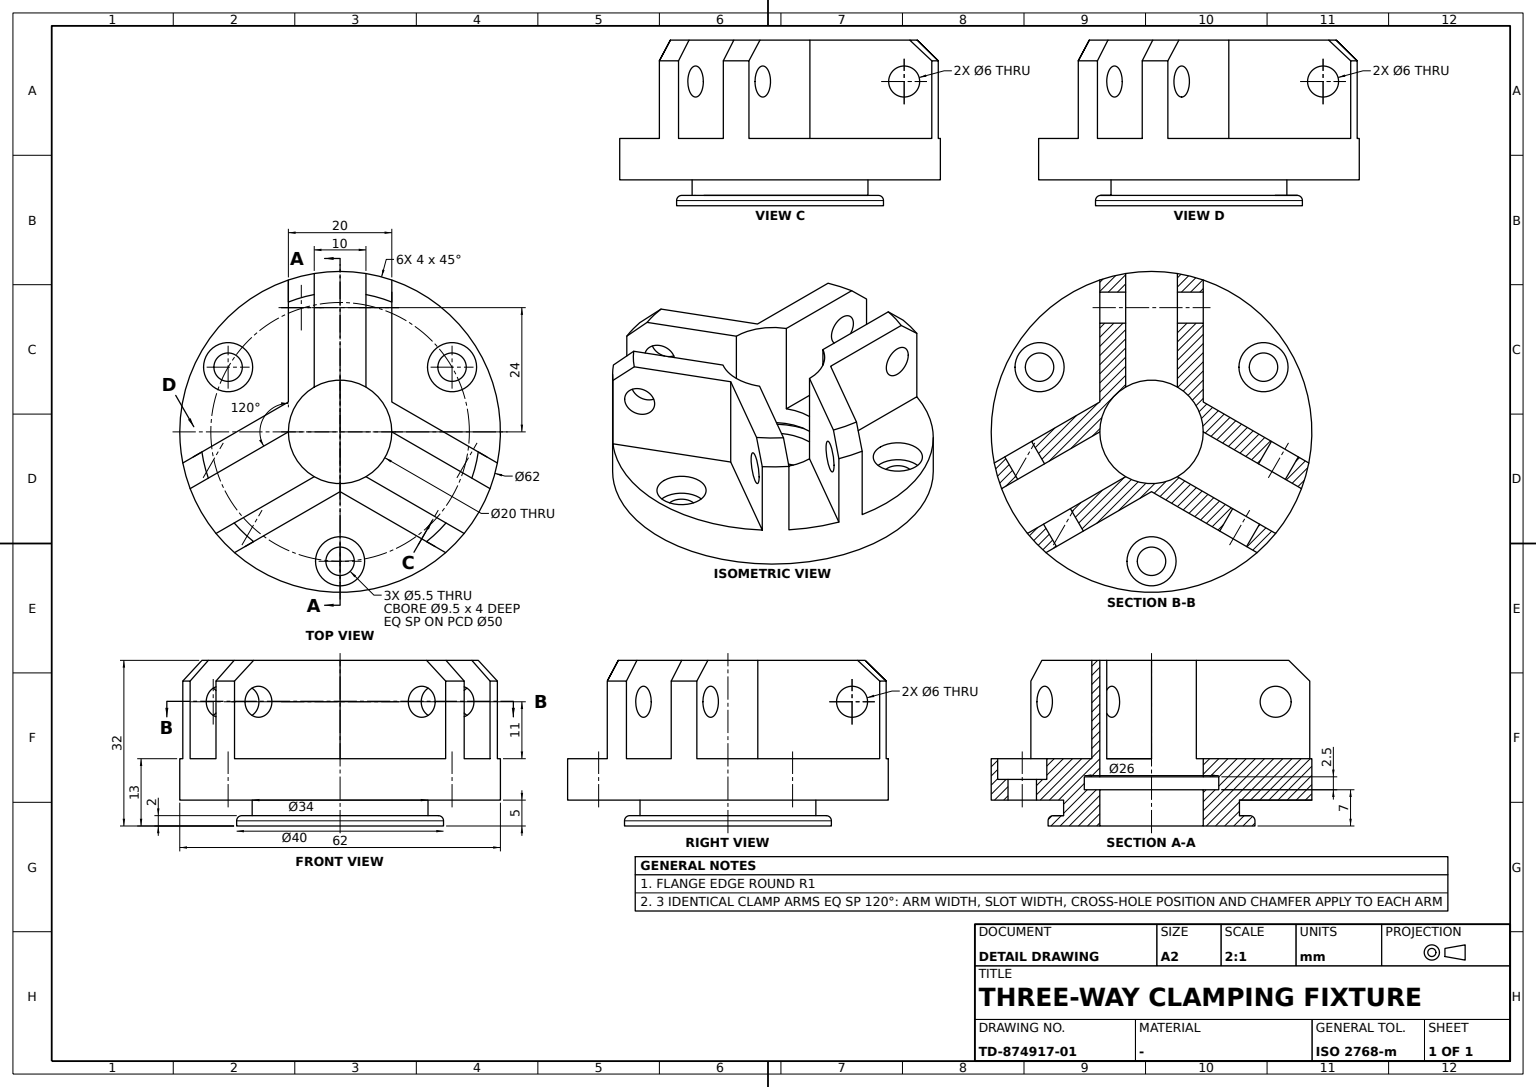
ISO-10303-21;
HEADER;
FILE_DESCRIPTION((''),'2;1');
FILE_NAME('','',(''),(''),'','','');
FILE_SCHEMA(('AUTOMOTIVE_DESIGN'));
ENDSEC;
DATA;
#1=APPLICATION_CONTEXT('');
#2=PRODUCT_CONTEXT('',#1,'mechanical');
#3=PRODUCT('','','',(#2));
#4=PRODUCT_DEFINITION_FORMATION('','',#3);
#5=PRODUCT_DEFINITION_CONTEXT('',#1,'design');
#6=PRODUCT_DEFINITION('','',#4,#5);
#7=PRODUCT_DEFINITION_SHAPE('','',#6);
#8=(LENGTH_UNIT()NAMED_UNIT(*)SI_UNIT(.MILLI.,.METRE.));
#9=(NAMED_UNIT(*)PLANE_ANGLE_UNIT()SI_UNIT($,.RADIAN.));
#10=(NAMED_UNIT(*)SI_UNIT($,.STERADIAN.)SOLID_ANGLE_UNIT());
#11=UNCERTAINTY_MEASURE_WITH_UNIT(LENGTH_MEASURE(0.005),#8,'distance_accuracy_value','');
#12=(GEOMETRIC_REPRESENTATION_CONTEXT(3)GLOBAL_UNCERTAINTY_ASSIGNED_CONTEXT((#11))GLOBAL_UNIT_ASSIGNED_CONTEXT((#8,#9,#10))REPRESENTATION_CONTEXT('',''));
#13=CARTESIAN_POINT('',(-26.400635,12.5,13.));
#14=VERTEX_POINT('',#13);
#15=CARTESIAN_POINT('',(-21.650635,12.5,13.));
#16=DIRECTION('',(0.,0.,-1.));
#17=DIRECTION('',(-1.,0.,0.));
#18=AXIS2_PLACEMENT_3D('',#15,#16,#17);
#19=CIRCLE('',#18,4.75);
#20=EDGE_CURVE('',#14,#14,#19,.T.);
#21=ORIENTED_EDGE('',*,*,#20,.F.);
#22=EDGE_LOOP('',(#21));
#23=FACE_BOUND('',#22,.T.);
#24=CARTESIAN_POINT('',(-26.400635,12.5,9.));
#25=VERTEX_POINT('',#24);
#26=CARTESIAN_POINT('',(-21.650635,12.5,9.));
#27=AXIS2_PLACEMENT_3D('',#26,#16,#17);
#28=CIRCLE('',#27,4.75);
#29=EDGE_CURVE('',#25,#25,#28,.F.);
#30=ORIENTED_EDGE('',*,*,#29,.F.);
#31=EDGE_LOOP('',(#30));
#32=FACE_BOUND('',#31,.T.);
#33=CYLINDRICAL_SURFACE('',#18,4.75);
#34=ADVANCED_FACE('',(#23,#32),#33,.F.);
#35=CARTESIAN_POINT('',(-24.400635,12.5,9.));
#36=VERTEX_POINT('',#35);
#37=CIRCLE('',#27,2.75);
#38=EDGE_CURVE('',#36,#36,#37,.F.);
#39=ORIENTED_EDGE('',*,*,#38,.T.);
#40=EDGE_LOOP('',(#39));
#41=FACE_BOUND('',#40,.T.);
#42=CARTESIAN_POINT('',(-18.900635,12.5,5.));
#43=VERTEX_POINT('',#42);
#44=CARTESIAN_POINT('',(-21.650635,12.5,5.));
#45=DIRECTION('',(0.,0.,1.));
#46=DIRECTION('',(1.,0.,0.));
#47=AXIS2_PLACEMENT_3D('',#44,#45,#46);
#48=CIRCLE('',#47,2.75);
#49=EDGE_CURVE('',#43,#43,#48,.F.);
#50=ORIENTED_EDGE('',*,*,#49,.T.);
#51=EDGE_LOOP('',(#50));
#52=FACE_BOUND('',#51,.T.);
#53=CARTESIAN_POINT('',(-21.650635,12.5,-28.837261));
#54=AXIS2_PLACEMENT_3D('',#53,#16,#17);
#55=CYLINDRICAL_SURFACE('',#54,2.75);
#56=ADVANCED_FACE('',(#41,#52),#55,.F.);
#57=CARTESIAN_POINT('',(5.,26.532998,32.));
#58=VERTEX_POINT('',#57);
#59=CARTESIAN_POINT('',(5.,8.660254,32.));
#60=VERTEX_POINT('',#59);
#61=CARTESIAN_POINT('',(5.,30.594117,32.));
#62=DIRECTION('',(0.,-1.,0.));
#63=VECTOR('',#62,1000.);
#64=LINE('',#61,#63);
#65=EDGE_CURVE('',#58,#60,#64,.T.);
#66=ORIENTED_EDGE('',*,*,#65,.T.);
#67=CARTESIAN_POINT('',(10.,0.,32.));
#68=VERTEX_POINT('',#67);
#69=CARTESIAN_POINT('',(0.,0.,32.));
#70=AXIS2_PLACEMENT_3D('',#69,#45,#46);
#71=CIRCLE('',#70,10.);
#72=EDGE_CURVE('',#68,#60,#71,.T.);
#73=ORIENTED_EDGE('',*,*,#72,.F.);
#74=CARTESIAN_POINT('',(25.478251,-8.936372,32.));
#75=VERTEX_POINT('',#74);
#76=CARTESIAN_POINT('',(5.,2.886751,32.));
#77=DIRECTION('',(0.866025404,-0.5,0.));
#78=VECTOR('',#77,1000.);
#79=LINE('',#76,#78);
#80=EDGE_CURVE('',#68,#75,#79,.T.);
#81=ORIENTED_EDGE('',*,*,#80,.T.);
#82=CARTESIAN_POINT('',(26.719807,-3.879682,32.));
#83=VERTEX_POINT('',#82);
#84=CIRCLE('',#70,27.);
#85=EDGE_CURVE('',#75,#83,#84,.T.);
#86=ORIENTED_EDGE('',*,*,#85,.T.);
#87=CARTESIAN_POINT('',(10.,5.773503,32.));
#88=VERTEX_POINT('',#87);
#89=CARTESIAN_POINT('',(30.411612,-6.011147,32.));
#90=DIRECTION('',(-0.866025404,0.5,0.));
#91=VECTOR('',#90,1000.);
#92=LINE('',#89,#91);
#93=EDGE_CURVE('',#83,#88,#92,.T.);
#94=ORIENTED_EDGE('',*,*,#93,.T.);
#95=CARTESIAN_POINT('',(10.,25.079872,32.));
#96=VERTEX_POINT('',#95);
#97=DIRECTION('',(0.,1.,0.));
#98=VECTOR('',#97,1000.);
#99=LINE('',#87,#98);
#100=EDGE_CURVE('',#88,#96,#99,.T.);
#101=ORIENTED_EDGE('',*,*,#100,.T.);
#102=EDGE_CURVE('',#96,#58,#84,.T.);
#103=ORIENTED_EDGE('',*,*,#102,.T.);
#104=EDGE_LOOP('',(#66,#73,#81,#86,#94,#101,#103));
#105=FACE_BOUND('',#104,.T.);
#106=PLANE('',#70);
#107=ADVANCED_FACE('',(#105),#106,.T.);
#108=CARTESIAN_POINT('',(-4.75,-25.,13.));
#109=VERTEX_POINT('',#108);
#110=CARTESIAN_POINT('',(0.,-25.,13.));
#111=AXIS2_PLACEMENT_3D('',#110,#16,#17);
#112=CIRCLE('',#111,4.75);
#113=EDGE_CURVE('',#109,#109,#112,.T.);
#114=ORIENTED_EDGE('',*,*,#113,.T.);
#115=EDGE_LOOP('',(#114));
#116=FACE_BOUND('',#115,.T.);
#117=CARTESIAN_POINT('',(20.411612,-23.331655,13.));
#118=VERTEX_POINT('',#117);
#119=CARTESIAN_POINT('',(-20.411612,-23.331655,13.));
#120=VERTEX_POINT('',#119);
#121=CARTESIAN_POINT('',(0.,0.,13.));
#122=AXIS2_PLACEMENT_3D('',#121,#16,#17);
#123=CIRCLE('',#122,31.);
#124=EDGE_CURVE('',#118,#120,#123,.T.);
#125=ORIENTED_EDGE('',*,*,#124,.F.);
#126=CARTESIAN_POINT('',(0.,-11.547005,13.));
#127=VERTEX_POINT('',#126);
#128=CARTESIAN_POINT('',(-9.330127,-6.160254,13.));
#129=LINE('',#128,#91);
#130=EDGE_CURVE('',#127,#118,#129,.F.);
#131=ORIENTED_EDGE('',*,*,#130,.F.);
#132=CARTESIAN_POINT('',(9.330127,-6.160254,13.));
#133=DIRECTION('',(-0.866025404,-0.5,0.));
#134=VECTOR('',#133,1000.);
#135=LINE('',#132,#134);
#136=EDGE_CURVE('',#120,#127,#135,.F.);
#137=ORIENTED_EDGE('',*,*,#136,.F.);
#138=EDGE_LOOP('',(#125,#131,#137));
#139=FACE_BOUND('',#138,.T.);
#140=CARTESIAN_POINT('',(0.,10.,13.));
#141=AXIS2_PLACEMENT_3D('',#140,#16,#17);
#142=PLANE('',#141);
#143=ADVANCED_FACE('',(#116,#139),#142,.F.);
#144=CARTESIAN_POINT('',(-20.,0.,0.));
#145=VERTEX_POINT('',#144);
#146=CARTESIAN_POINT('',(0.,0.,0.));
#147=AXIS2_PLACEMENT_3D('',#146,#16,#17);
#148=CIRCLE('',#147,20.);
#149=EDGE_CURVE('',#145,#145,#148,.T.);
#150=ORIENTED_EDGE('',*,*,#149,.F.);
#151=EDGE_LOOP('',(#150));
#152=FACE_BOUND('',#151,.T.);
#153=CARTESIAN_POINT('',(-20.,0.,1.));
#154=VERTEX_POINT('',#153);
#155=CARTESIAN_POINT('',(0.,0.,1.));
#156=AXIS2_PLACEMENT_3D('',#155,#16,#17);
#157=CIRCLE('',#156,20.);
#158=EDGE_CURVE('',#154,#154,#157,.T.);
#159=ORIENTED_EDGE('',*,*,#158,.T.);
#160=EDGE_LOOP('',(#159));
#161=FACE_BOUND('',#160,.T.);
#162=CYLINDRICAL_SURFACE('',#147,20.);
#163=ADVANCED_FACE('',(#152,#161),#162,.T.);
#164=CARTESIAN_POINT('',(-23.995283,-19.627186,13.));
#165=VERTEX_POINT('',#164);
#166=CARTESIAN_POINT('',(-28.995283,-10.966932,13.));
#167=VERTEX_POINT('',#166);
#168=EDGE_CURVE('',#165,#167,#123,.T.);
#169=ORIENTED_EDGE('',*,*,#168,.F.);
#170=CARTESIAN_POINT('',(-5.,-8.660254,13.));
#171=VERTEX_POINT('',#170);
#172=CARTESIAN_POINT('',(6.830127,-1.830127,13.));
#173=DIRECTION('',(0.866025404,0.5,0.));
#174=VECTOR('',#173,1000.);
#175=LINE('',#172,#174);
#176=EDGE_CURVE('',#171,#165,#175,.F.);
#177=ORIENTED_EDGE('',*,*,#176,.F.);
#178=CARTESIAN_POINT('',(-10.,0.,13.));
#179=VERTEX_POINT('',#178);
#180=CIRCLE('',#122,10.);
#181=EDGE_CURVE('',#171,#179,#180,.T.);
#182=ORIENTED_EDGE('',*,*,#181,.T.);
#183=CARTESIAN_POINT('',(1.830127,6.830127,13.));
#184=LINE('',#183,#134);
#185=EDGE_CURVE('',#167,#179,#184,.F.);
#186=ORIENTED_EDGE('',*,*,#185,.F.);
#187=EDGE_LOOP('',(#169,#177,#182,#186));
#188=FACE_BOUND('',#187,.T.);
#189=ADVANCED_FACE('',(#188),#142,.F.);
#190=CARTESIAN_POINT('',(-17.,0.,5.));
#191=VERTEX_POINT('',#190);
#192=CARTESIAN_POINT('',(0.,0.,5.));
#193=AXIS2_PLACEMENT_3D('',#192,#16,#17);
#194=CIRCLE('',#193,17.);
#195=EDGE_CURVE('',#191,#191,#194,.T.);
#196=ORIENTED_EDGE('',*,*,#195,.F.);
#197=EDGE_LOOP('',(#196));
#198=FACE_BOUND('',#197,.T.);
#199=CARTESIAN_POINT('',(-31.,0.,5.));
#200=VERTEX_POINT('',#199);
#201=CIRCLE('',#193,31.);
#202=EDGE_CURVE('',#200,#200,#201,.T.);
#203=ORIENTED_EDGE('',*,*,#202,.T.);
#204=EDGE_LOOP('',(#203));
#205=FACE_BOUND('',#204,.T.);
#206=ORIENTED_EDGE('',*,*,#49,.F.);
#207=EDGE_LOOP('',(#206));
#208=FACE_BOUND('',#207,.T.);
#209=CARTESIAN_POINT('',(2.75,-25.,5.));
#210=VERTEX_POINT('',#209);
#211=CARTESIAN_POINT('',(0.,-25.,5.));
#212=AXIS2_PLACEMENT_3D('',#211,#45,#46);
#213=CIRCLE('',#212,2.75);
#214=EDGE_CURVE('',#210,#210,#213,.F.);
#215=ORIENTED_EDGE('',*,*,#214,.F.);
#216=EDGE_LOOP('',(#215));
#217=FACE_BOUND('',#216,.T.);
#218=CARTESIAN_POINT('',(24.400635,12.5,5.));
#219=VERTEX_POINT('',#218);
#220=CARTESIAN_POINT('',(21.650635,12.5,5.));
#221=AXIS2_PLACEMENT_3D('',#220,#45,#46);
#222=CIRCLE('',#221,2.75);
#223=EDGE_CURVE('',#219,#219,#222,.F.);
#224=ORIENTED_EDGE('',*,*,#223,.F.);
#225=EDGE_LOOP('',(#224));
#226=FACE_BOUND('',#225,.T.);
#227=CARTESIAN_POINT('',(0.,31.,5.));
#228=AXIS2_PLACEMENT_3D('',#227,#45,#46);
#229=PLANE('',#228);
#230=ADVANCED_FACE('',(#198,#205,#208,#217,#226),#229,.F.);
#231=CARTESIAN_POINT('',(-20.882686,-17.830127,24.));
#232=VERTEX_POINT('',#231);
#233=CARTESIAN_POINT('',(-18.28461,-16.330127,24.));
#234=DIRECTION('',(-0.5,0.866025404,0.));
#235=AXIS2_PLACEMENT_3D('',#233,#234,#133);
#236=CIRCLE('',#235,3.);
#237=EDGE_CURVE('',#232,#232,#236,.T.);
#238=ORIENTED_EDGE('',*,*,#237,.T.);
#239=EDGE_LOOP('',(#238));
#240=FACE_BOUND('',#239,.T.);
#241=CARTESIAN_POINT('',(-18.382686,-22.160254,24.));
#242=VERTEX_POINT('',#241);
#243=CARTESIAN_POINT('',(-15.78461,-20.660254,24.));
#244=AXIS2_PLACEMENT_3D('',#243,#234,#133);
#245=CIRCLE('',#244,3.);
#246=EDGE_CURVE('',#242,#242,#245,.T.);
#247=ORIENTED_EDGE('',*,*,#246,.F.);
#248=EDGE_LOOP('',(#247));
#249=FACE_BOUND('',#248,.T.);
#250=CYLINDRICAL_SURFACE('',#244,3.);
#251=ADVANCED_FACE('',(#240,#249),#250,.F.);
#252=CARTESIAN_POINT('',(28.382686,-4.839746,24.));
#253=VERTEX_POINT('',#252);
#254=CARTESIAN_POINT('',(25.78461,-3.339746,24.));
#255=DIRECTION('',(-0.5,-0.866025404,0.));
#256=AXIS2_PLACEMENT_3D('',#254,#255,#77);
#257=CIRCLE('',#256,3.);
#258=EDGE_CURVE('',#253,#253,#257,.T.);
#259=ORIENTED_EDGE('',*,*,#258,.T.);
#260=EDGE_LOOP('',(#259));
#261=FACE_BOUND('',#260,.T.);
#262=CARTESIAN_POINT('',(30.411612,-6.011147,13.));
#263=VERTEX_POINT('',#262);
#264=CARTESIAN_POINT('',(10.,5.773503,13.));
#265=VERTEX_POINT('',#264);
#266=CARTESIAN_POINT('',(0.669873,11.160254,13.));
#267=LINE('',#266,#78);
#268=EDGE_CURVE('',#263,#265,#267,.F.);
#269=ORIENTED_EDGE('',*,*,#268,.T.);
#270=CARTESIAN_POINT('',(10.,5.773503,5.));
#271=VECTOR('',#45,1000.);
#272=LINE('',#270,#271);
#273=EDGE_CURVE('',#265,#88,#272,.T.);
#274=ORIENTED_EDGE('',*,*,#273,.T.);
#275=ORIENTED_EDGE('',*,*,#93,.F.);
#276=CARTESIAN_POINT('',(30.411612,-6.011147,28.));
#277=VERTEX_POINT('',#276);
#278=CARTESIAN_POINT('',(27.956231,-4.593532,30.673832));
#279=CARTESIAN_POINT('',(29.186037,-5.303561,29.339519));
#280=B_SPLINE_CURVE_WITH_KNOTS('',3,(#82,#278,#279,#276),.UNSPECIFIED.,.F.,.F.,(4,4),(0.,0.00584573),.UNSPECIFIED.);
#281=EDGE_CURVE('',#83,#277,#280,.T.);
#282=ORIENTED_EDGE('',*,*,#281,.T.);
#283=CARTESIAN_POINT('',(30.411612,-6.011147,5.));
#284=LINE('',#283,#271);
#285=EDGE_CURVE('',#263,#277,#284,.T.);
#286=ORIENTED_EDGE('',*,*,#285,.F.);
#287=EDGE_LOOP('',(#269,#274,#275,#282,#286));
#288=FACE_BOUND('',#287,.T.);
#289=DIRECTION('',(0.5,0.866025404,0.));
#290=AXIS2_PLACEMENT_3D('',#283,#289,#90);
#291=PLANE('',#290);
#292=ADVANCED_FACE('',(#261,#288),#291,.T.);
#293=CARTESIAN_POINT('',(15.686533,-14.830127,24.));
#294=VERTEX_POINT('',#293);
#295=CARTESIAN_POINT('',(18.28461,-16.330127,24.));
#296=AXIS2_PLACEMENT_3D('',#295,#289,#90);
#297=CIRCLE('',#296,3.);
#298=EDGE_CURVE('',#294,#294,#297,.T.);
#299=ORIENTED_EDGE('',*,*,#298,.F.);
#300=EDGE_LOOP('',(#299));
#301=FACE_BOUND('',#300,.T.);
#302=CARTESIAN_POINT('',(20.478251,-17.596626,32.));
#303=VERTEX_POINT('',#302);
#304=CARTESIAN_POINT('',(23.995283,-19.627186,28.));
#305=VERTEX_POINT('',#304);
#306=CARTESIAN_POINT('',(21.651913,-18.27424,30.668212));
#307=CARTESIAN_POINT('',(22.824084,-18.950994,29.334677));
#308=B_SPLINE_CURVE_WITH_KNOTS('',3,(#302,#306,#307,#304),.UNSPECIFIED.,.F.,.F.,(4,4),(0.,0.005700236),.UNSPECIFIED.);
#309=EDGE_CURVE('',#303,#305,#308,.T.);
#310=ORIENTED_EDGE('',*,*,#309,.T.);
#311=CARTESIAN_POINT('',(23.995283,-19.627186,13.));
#312=VERTEX_POINT('',#311);
#313=CARTESIAN_POINT('',(23.995283,-19.627186,5.));
#314=LINE('',#313,#271);
#315=EDGE_CURVE('',#312,#305,#314,.T.);
#316=ORIENTED_EDGE('',*,*,#315,.F.);
#317=CARTESIAN_POINT('',(5.,-8.660254,13.));
#318=VERTEX_POINT('',#317);
#319=CARTESIAN_POINT('',(-6.830127,-1.830127,13.));
#320=LINE('',#319,#78);
#321=EDGE_CURVE('',#312,#318,#320,.F.);
#322=ORIENTED_EDGE('',*,*,#321,.T.);
#323=CARTESIAN_POINT('',(5.,-8.660254,32.));
#324=VERTEX_POINT('',#323);
#325=CARTESIAN_POINT('',(5.,-8.660254,-15.));
#326=LINE('',#325,#271);
#327=EDGE_CURVE('',#318,#324,#326,.T.);
#328=ORIENTED_EDGE('',*,*,#327,.T.);
#329=CARTESIAN_POINT('',(23.995283,-19.627186,32.));
#330=LINE('',#329,#91);
#331=EDGE_CURVE('',#303,#324,#330,.T.);
#332=ORIENTED_EDGE('',*,*,#331,.F.);
#333=EDGE_LOOP('',(#310,#316,#322,#328,#332));
#334=FACE_BOUND('',#333,.T.);
#335=AXIS2_PLACEMENT_3D('',#313,#289,#90);
#336=PLANE('',#335);
#337=ADVANCED_FACE('',(#301,#334),#336,.T.);
#338=CARTESIAN_POINT('',(-25.478251,-8.936372,32.));
#339=VERTEX_POINT('',#338);
#340=CARTESIAN_POINT('',(-10.,0.,32.));
#341=VERTEX_POINT('',#340);
#342=CARTESIAN_POINT('',(-28.995283,-10.966932,32.));
#343=LINE('',#342,#174);
#344=EDGE_CURVE('',#339,#341,#343,.T.);
#345=ORIENTED_EDGE('',*,*,#344,.F.);
#346=CARTESIAN_POINT('',(-28.995283,-10.966932,28.));
#347=VERTEX_POINT('',#346);
#348=CARTESIAN_POINT('',(-26.651913,-9.613986,30.668212));
#349=CARTESIAN_POINT('',(-27.824084,-10.29074,29.334677));
#350=B_SPLINE_CURVE_WITH_KNOTS('',3,(#338,#348,#349,#346),.UNSPECIFIED.,.F.,.F.,(4,4),(0.,0.005700236),.UNSPECIFIED.);
#351=EDGE_CURVE('',#339,#347,#350,.T.);
#352=ORIENTED_EDGE('',*,*,#351,.T.);
#353=CARTESIAN_POINT('',(-28.995283,-10.966932,5.));
#354=LINE('',#353,#271);
#355=EDGE_CURVE('',#167,#347,#354,.T.);
#356=ORIENTED_EDGE('',*,*,#355,.F.);
#357=ORIENTED_EDGE('',*,*,#185,.T.);
#358=CARTESIAN_POINT('',(-10.,0.,-15.));
#359=LINE('',#358,#271);
#360=EDGE_CURVE('',#179,#341,#359,.T.);
#361=ORIENTED_EDGE('',*,*,#360,.T.);
#362=EDGE_LOOP('',(#345,#352,#356,#357,#361));
#363=FACE_BOUND('',#362,.T.);
#364=CARTESIAN_POINT('',(-20.686533,-6.169873,24.));
#365=VERTEX_POINT('',#364);
#366=CARTESIAN_POINT('',(-23.28461,-7.669873,24.));
#367=DIRECTION('',(0.5,-0.866025404,0.));
#368=AXIS2_PLACEMENT_3D('',#366,#367,#173);
#369=CIRCLE('',#368,3.);
#370=EDGE_CURVE('',#365,#365,#369,.T.);
#371=ORIENTED_EDGE('',*,*,#370,.F.);
#372=EDGE_LOOP('',(#371));
#373=FACE_BOUND('',#372,.T.);
#374=AXIS2_PLACEMENT_3D('',#353,#367,#173);
#375=PLANE('',#374);
#376=ADVANCED_FACE('',(#363,#373),#375,.T.);
#377=CARTESIAN_POINT('',(-30.411612,-6.011147,28.));
#378=VERTEX_POINT('',#377);
#379=CARTESIAN_POINT('',(-26.719807,-3.879682,32.));
#380=VERTEX_POINT('',#379);
#381=CARTESIAN_POINT('',(-29.186037,-5.303561,29.339519));
#382=CARTESIAN_POINT('',(-27.956231,-4.593532,30.673832));
#383=B_SPLINE_CURVE_WITH_KNOTS('',3,(#377,#381,#382,#379),.UNSPECIFIED.,.F.,.F.,(4,4),(0.,0.00584573),.UNSPECIFIED.);
#384=EDGE_CURVE('',#378,#380,#383,.T.);
#385=ORIENTED_EDGE('',*,*,#384,.F.);
#386=CARTESIAN_POINT('',(0.,0.,28.));
#387=AXIS2_PLACEMENT_3D('',#386,#45,#46);
#388=CIRCLE('',#387,31.);
#389=EDGE_CURVE('',#347,#378,#388,.F.);
#390=ORIENTED_EDGE('',*,*,#389,.F.);
#391=ORIENTED_EDGE('',*,*,#351,.F.);
#392=EDGE_CURVE('',#380,#339,#84,.T.);
#393=ORIENTED_EDGE('',*,*,#392,.F.);
#394=EDGE_LOOP('',(#385,#390,#391,#393));
#395=FACE_BOUND('',#394,.T.);
#396=AXIS2_PLACEMENT_3D('',#69,#16,#17);
#397=CONICAL_SURFACE('',#396,27.,0.785398163);
#398=ADVANCED_FACE('',(#395),#397,.T.);
#399=CARTESIAN_POINT('',(28.995283,-10.966932,28.));
#400=VERTEX_POINT('',#399);
#401=CARTESIAN_POINT('',(27.824084,-10.29074,29.334677));
#402=CARTESIAN_POINT('',(26.651913,-9.613986,30.668212));
#403=B_SPLINE_CURVE_WITH_KNOTS('',3,(#399,#401,#402,#74),.UNSPECIFIED.,.F.,.F.,(4,4),(0.,0.005700236),.UNSPECIFIED.);
#404=EDGE_CURVE('',#400,#75,#403,.T.);
#405=ORIENTED_EDGE('',*,*,#404,.T.);
#406=ORIENTED_EDGE('',*,*,#80,.F.);
#407=CARTESIAN_POINT('',(10.,0.,13.));
#408=VERTEX_POINT('',#407);
#409=CARTESIAN_POINT('',(10.,0.,-15.));
#410=LINE('',#409,#271);
#411=EDGE_CURVE('',#68,#408,#410,.F.);
#412=ORIENTED_EDGE('',*,*,#411,.T.);
#413=CARTESIAN_POINT('',(28.995283,-10.966932,13.));
#414=VERTEX_POINT('',#413);
#415=CARTESIAN_POINT('',(-1.830127,6.830127,13.));
#416=LINE('',#415,#91);
#417=EDGE_CURVE('',#408,#414,#416,.F.);
#418=ORIENTED_EDGE('',*,*,#417,.T.);
#419=CARTESIAN_POINT('',(28.995283,-10.966932,5.));
#420=LINE('',#419,#271);
#421=EDGE_CURVE('',#414,#400,#420,.T.);
#422=ORIENTED_EDGE('',*,*,#421,.T.);
#423=EDGE_LOOP('',(#405,#406,#412,#418,#422));
#424=FACE_BOUND('',#423,.T.);
#425=CARTESIAN_POINT('',(25.882686,-9.169873,24.));
#426=VERTEX_POINT('',#425);
#427=CARTESIAN_POINT('',(23.28461,-7.669873,24.));
#428=AXIS2_PLACEMENT_3D('',#427,#255,#77);
#429=CIRCLE('',#428,3.);
#430=EDGE_CURVE('',#426,#426,#429,.T.);
#431=ORIENTED_EDGE('',*,*,#430,.F.);
#432=EDGE_LOOP('',(#431));
#433=FACE_BOUND('',#432,.T.);
#434=CARTESIAN_POINT('',(5.,2.886751,5.));
#435=AXIS2_PLACEMENT_3D('',#434,#255,#77);
#436=PLANE('',#435);
#437=ADVANCED_FACE('',(#424,#433),#436,.T.);
#438=ORIENTED_EDGE('',*,*,#214,.T.);
#439=EDGE_LOOP('',(#438));
#440=FACE_BOUND('',#439,.T.);
#441=CARTESIAN_POINT('',(-2.75,-25.,9.));
#442=VERTEX_POINT('',#441);
#443=CARTESIAN_POINT('',(0.,-25.,9.));
#444=AXIS2_PLACEMENT_3D('',#443,#16,#17);
#445=CIRCLE('',#444,2.75);
#446=EDGE_CURVE('',#442,#442,#445,.F.);
#447=ORIENTED_EDGE('',*,*,#446,.T.);
#448=EDGE_LOOP('',(#447));
#449=FACE_BOUND('',#448,.T.);
#450=CARTESIAN_POINT('',(0.,-25.,-28.837261));
#451=AXIS2_PLACEMENT_3D('',#450,#16,#17);
#452=CYLINDRICAL_SURFACE('',#451,2.75);
#453=ADVANCED_FACE('',(#440,#449),#452,.F.);
#454=CARTESIAN_POINT('',(-17.,0.,2.));
#455=VERTEX_POINT('',#454);
#456=CARTESIAN_POINT('',(0.,0.,2.));
#457=AXIS2_PLACEMENT_3D('',#456,#16,#17);
#458=CIRCLE('',#457,17.);
#459=EDGE_CURVE('',#455,#455,#458,.T.);
#460=ORIENTED_EDGE('',*,*,#459,.F.);
#461=EDGE_LOOP('',(#460));
#462=FACE_BOUND('',#461,.T.);
#463=ORIENTED_EDGE('',*,*,#195,.T.);
#464=EDGE_LOOP('',(#463));
#465=FACE_BOUND('',#464,.T.);
#466=CYLINDRICAL_SURFACE('',#147,17.);
#467=ADVANCED_FACE('',(#462,#465),#466,.T.);
#468=CARTESIAN_POINT('',(16.900635,12.5,9.));
#469=VERTEX_POINT('',#468);
#470=CARTESIAN_POINT('',(21.650635,12.5,9.));
#471=AXIS2_PLACEMENT_3D('',#470,#16,#17);
#472=CIRCLE('',#471,4.75);
#473=EDGE_CURVE('',#469,#469,#472,.F.);
#474=ORIENTED_EDGE('',*,*,#473,.F.);
#475=EDGE_LOOP('',(#474));
#476=FACE_BOUND('',#475,.T.);
#477=CARTESIAN_POINT('',(16.900635,12.5,13.));
#478=VERTEX_POINT('',#477);
#479=CARTESIAN_POINT('',(21.650635,12.5,13.));
#480=AXIS2_PLACEMENT_3D('',#479,#16,#17);
#481=CIRCLE('',#480,4.75);
#482=EDGE_CURVE('',#478,#478,#481,.T.);
#483=ORIENTED_EDGE('',*,*,#482,.F.);
#484=EDGE_LOOP('',(#483));
#485=FACE_BOUND('',#484,.T.);
#486=CYLINDRICAL_SURFACE('',#480,4.75);
#487=ADVANCED_FACE('',(#476,#485),#486,.F.);
#488=CARTESIAN_POINT('',(10.,0.,9.5));
#489=VERTEX_POINT('',#488);
#490=CARTESIAN_POINT('',(0.,0.,9.5));
#491=AXIS2_PLACEMENT_3D('',#490,#45,#46);
#492=CIRCLE('',#491,10.);
#493=EDGE_CURVE('',#489,#489,#492,.F.);
#494=ORIENTED_EDGE('',*,*,#493,.F.);
#495=EDGE_LOOP('',(#494));
#496=FACE_BOUND('',#495,.T.);
#497=CARTESIAN_POINT('',(13.,0.,9.5));
#498=VERTEX_POINT('',#497);
#499=CIRCLE('',#491,13.);
#500=EDGE_CURVE('',#498,#498,#499,.F.);
#501=ORIENTED_EDGE('',*,*,#500,.T.);
#502=EDGE_LOOP('',(#501));
#503=FACE_BOUND('',#502,.T.);
#504=PLANE('',#491);
#505=ADVANCED_FACE('',(#496,#503),#504,.F.);
#506=CARTESIAN_POINT('',(-10.,24.,21.));
#507=VERTEX_POINT('',#506);
#508=CARTESIAN_POINT('',(-10.,24.,24.));
#509=AXIS2_PLACEMENT_3D('',#508,#46,#16);
#510=CIRCLE('',#509,3.);
#511=EDGE_CURVE('',#507,#507,#510,.T.);
#512=ORIENTED_EDGE('',*,*,#511,.T.);
#513=EDGE_LOOP('',(#512));
#514=FACE_BOUND('',#513,.T.);
#515=CARTESIAN_POINT('',(-10.,25.079872,32.));
#516=VERTEX_POINT('',#515);
#517=CARTESIAN_POINT('',(-10.,29.342802,28.));
#518=VERTEX_POINT('',#517);
#519=CARTESIAN_POINT('',(-10.,26.507572,30.673832));
#520=CARTESIAN_POINT('',(-10.,27.92763,29.339519));
#521=B_SPLINE_CURVE_WITH_KNOTS('',3,(#515,#519,#520,#517),.UNSPECIFIED.,.F.,.F.,(4,4),(0.,0.00584573),.UNSPECIFIED.);
#522=EDGE_CURVE('',#516,#518,#521,.T.);
#523=ORIENTED_EDGE('',*,*,#522,.T.);
#524=CARTESIAN_POINT('',(-10.,29.342802,13.));
#525=VERTEX_POINT('',#524);
#526=CARTESIAN_POINT('',(-10.,29.342802,5.));
#527=LINE('',#526,#271);
#528=EDGE_CURVE('',#525,#518,#527,.T.);
#529=ORIENTED_EDGE('',*,*,#528,.F.);
#530=CARTESIAN_POINT('',(-10.,5.773503,13.));
#531=VERTEX_POINT('',#530);
#532=CARTESIAN_POINT('',(-10.,10.,13.));
#533=LINE('',#532,#98);
#534=EDGE_CURVE('',#525,#531,#533,.F.);
#535=ORIENTED_EDGE('',*,*,#534,.T.);
#536=CARTESIAN_POINT('',(-10.,5.773503,32.));
#537=VERTEX_POINT('',#536);
#538=CARTESIAN_POINT('',(-10.,5.773503,5.));
#539=LINE('',#538,#271);
#540=EDGE_CURVE('',#531,#537,#539,.T.);
#541=ORIENTED_EDGE('',*,*,#540,.T.);
#542=CARTESIAN_POINT('',(-10.,29.342802,32.));
#543=LINE('',#542,#63);
#544=EDGE_CURVE('',#516,#537,#543,.T.);
#545=ORIENTED_EDGE('',*,*,#544,.F.);
#546=EDGE_LOOP('',(#523,#529,#535,#541,#545));
#547=FACE_BOUND('',#546,.T.);
#548=AXIS2_PLACEMENT_3D('',#526,#17,#45);
#549=PLANE('',#548);
#550=ADVANCED_FACE('',(#514,#547),#549,.T.);
#551=ORIENTED_EDGE('',*,*,#246,.T.);
#552=EDGE_LOOP('',(#551));
#553=FACE_BOUND('',#552,.T.);
#554=CARTESIAN_POINT('',(-16.719807,-21.20019,32.));
#555=VERTEX_POINT('',#554);
#556=CARTESIAN_POINT('',(-20.411612,-23.331655,28.));
#557=VERTEX_POINT('',#556);
#558=CARTESIAN_POINT('',(-17.956231,-21.91404,30.673832));
#559=CARTESIAN_POINT('',(-19.186037,-22.624069,29.339519));
#560=B_SPLINE_CURVE_WITH_KNOTS('',3,(#554,#558,#559,#556),.UNSPECIFIED.,.F.,.F.,(4,4),(0.,0.00584573),.UNSPECIFIED.);
#561=EDGE_CURVE('',#555,#557,#560,.T.);
#562=ORIENTED_EDGE('',*,*,#561,.T.);
#563=CARTESIAN_POINT('',(-20.411612,-23.331655,5.));
#564=LINE('',#563,#271);
#565=EDGE_CURVE('',#120,#557,#564,.T.);
#566=ORIENTED_EDGE('',*,*,#565,.F.);
#567=ORIENTED_EDGE('',*,*,#136,.T.);
#568=CARTESIAN_POINT('',(0.,-11.547005,32.));
#569=VERTEX_POINT('',#568);
#570=CARTESIAN_POINT('',(0.,-11.547005,5.));
#571=LINE('',#570,#271);
#572=EDGE_CURVE('',#127,#569,#571,.T.);
#573=ORIENTED_EDGE('',*,*,#572,.T.);
#574=CARTESIAN_POINT('',(-20.411612,-23.331655,32.));
#575=LINE('',#574,#174);
#576=EDGE_CURVE('',#555,#569,#575,.T.);
#577=ORIENTED_EDGE('',*,*,#576,.F.);
#578=EDGE_LOOP('',(#562,#566,#567,#573,#577));
#579=FACE_BOUND('',#578,.T.);
#580=AXIS2_PLACEMENT_3D('',#563,#367,#173);
#581=PLANE('',#580);
#582=ADVANCED_FACE('',(#553,#579),#581,.T.);
#583=CARTESIAN_POINT('',(-5.,27.,24.));
#584=VERTEX_POINT('',#583);
#585=CARTESIAN_POINT('',(-5.,24.,24.));
#586=AXIS2_PLACEMENT_3D('',#585,#46,#97);
#587=CIRCLE('',#586,3.);
#588=EDGE_CURVE('',#584,#584,#587,.T.);
#589=ORIENTED_EDGE('',*,*,#588,.T.);
#590=EDGE_LOOP('',(#589));
#591=FACE_BOUND('',#590,.T.);
#592=ORIENTED_EDGE('',*,*,#511,.F.);
#593=EDGE_LOOP('',(#592));
#594=FACE_BOUND('',#593,.T.);
#595=CYLINDRICAL_SURFACE('',#509,3.);
#596=ADVANCED_FACE('',(#591,#594),#595,.F.);
#597=CARTESIAN_POINT('',(10.,0.,7.));
#598=VERTEX_POINT('',#597);
#599=CARTESIAN_POINT('',(0.,0.,7.));
#600=AXIS2_PLACEMENT_3D('',#599,#45,#46);
#601=CIRCLE('',#600,10.);
#602=EDGE_CURVE('',#598,#598,#601,.F.);
#603=ORIENTED_EDGE('',*,*,#602,.F.);
#604=EDGE_LOOP('',(#603));
#605=FACE_BOUND('',#604,.T.);
#606=CARTESIAN_POINT('',(-10.,0.,0.));
#607=VERTEX_POINT('',#606);
#608=CIRCLE('',#147,10.);
#609=EDGE_CURVE('',#607,#607,#608,.T.);
#610=ORIENTED_EDGE('',*,*,#609,.T.);
#611=EDGE_LOOP('',(#610));
#612=FACE_BOUND('',#611,.T.);
#613=CYLINDRICAL_SURFACE('',#147,10.);
#614=ADVANCED_FACE('',(#605,#612),#613,.F.);
#615=CARTESIAN_POINT('',(-5.,-8.660254,32.));
#616=VERTEX_POINT('',#615);
#617=CARTESIAN_POINT('',(-20.478251,-17.596626,32.));
#618=VERTEX_POINT('',#617);
#619=CARTESIAN_POINT('',(0.,-5.773503,32.));
#620=LINE('',#619,#134);
#621=EDGE_CURVE('',#616,#618,#620,.T.);
#622=ORIENTED_EDGE('',*,*,#621,.T.);
#623=EDGE_CURVE('',#618,#555,#84,.T.);
#624=ORIENTED_EDGE('',*,*,#623,.T.);
#625=ORIENTED_EDGE('',*,*,#576,.T.);
#626=CARTESIAN_POINT('',(16.719807,-21.20019,32.));
#627=VERTEX_POINT('',#626);
#628=LINE('',#568,#78);
#629=EDGE_CURVE('',#569,#627,#628,.T.);
#630=ORIENTED_EDGE('',*,*,#629,.T.);
#631=EDGE_CURVE('',#627,#303,#84,.T.);
#632=ORIENTED_EDGE('',*,*,#631,.T.);
#633=ORIENTED_EDGE('',*,*,#331,.T.);
#634=EDGE_CURVE('',#616,#324,#71,.T.);
#635=ORIENTED_EDGE('',*,*,#634,.F.);
#636=EDGE_LOOP('',(#622,#624,#625,#630,#632,#633,#635));
#637=FACE_BOUND('',#636,.T.);
#638=ADVANCED_FACE('',(#637),#106,.T.);
#639=CARTESIAN_POINT('',(-28.382686,-4.839746,24.));
#640=VERTEX_POINT('',#639);
#641=CARTESIAN_POINT('',(-25.78461,-3.339746,24.));
#642=AXIS2_PLACEMENT_3D('',#641,#234,#133);
#643=CIRCLE('',#642,3.);
#644=EDGE_CURVE('',#640,#640,#643,.T.);
#645=ORIENTED_EDGE('',*,*,#644,.F.);
#646=EDGE_LOOP('',(#645));
#647=FACE_BOUND('',#646,.T.);
#648=CARTESIAN_POINT('',(-30.411612,-6.011147,13.));
#649=VERTEX_POINT('',#648);
#650=CARTESIAN_POINT('',(-0.669873,11.160254,13.));
#651=LINE('',#650,#174);
#652=EDGE_CURVE('',#531,#649,#651,.F.);
#653=ORIENTED_EDGE('',*,*,#652,.T.);
#654=CARTESIAN_POINT('',(-30.411612,-6.011147,5.));
#655=LINE('',#654,#271);
#656=EDGE_CURVE('',#649,#378,#655,.T.);
#657=ORIENTED_EDGE('',*,*,#656,.T.);
#658=ORIENTED_EDGE('',*,*,#384,.T.);
#659=LINE('',#536,#134);
#660=EDGE_CURVE('',#537,#380,#659,.T.);
#661=ORIENTED_EDGE('',*,*,#660,.F.);
#662=ORIENTED_EDGE('',*,*,#540,.F.);
#663=EDGE_LOOP('',(#653,#657,#658,#661,#662));
#664=FACE_BOUND('',#663,.T.);
#665=AXIS2_PLACEMENT_3D('',#538,#234,#133);
#666=PLANE('',#665);
#667=ADVANCED_FACE('',(#647,#664),#666,.T.);
#668=ORIENTED_EDGE('',*,*,#20,.T.);
#669=EDGE_LOOP('',(#668));
#670=FACE_BOUND('',#669,.T.);
#671=ORIENTED_EDGE('',*,*,#534,.F.);
#672=EDGE_CURVE('',#649,#525,#123,.T.);
#673=ORIENTED_EDGE('',*,*,#672,.F.);
#674=ORIENTED_EDGE('',*,*,#652,.F.);
#675=EDGE_LOOP('',(#671,#673,#674));
#676=FACE_BOUND('',#675,.T.);
#677=ADVANCED_FACE('',(#670,#676),#142,.F.);
#678=CARTESIAN_POINT('',(-4.75,-25.,9.));
#679=VERTEX_POINT('',#678);
#680=CIRCLE('',#444,4.75);
#681=EDGE_CURVE('',#679,#679,#680,.F.);
#682=ORIENTED_EDGE('',*,*,#681,.F.);
#683=EDGE_LOOP('',(#682));
#684=FACE_BOUND('',#683,.T.);
#685=ORIENTED_EDGE('',*,*,#113,.F.);
#686=EDGE_LOOP('',(#685));
#687=FACE_BOUND('',#686,.T.);
#688=CYLINDRICAL_SURFACE('',#111,4.75);
#689=ADVANCED_FACE('',(#684,#687),#688,.F.);
#690=CARTESIAN_POINT('',(-5.,8.660254,32.));
#691=VERTEX_POINT('',#690);
#692=CARTESIAN_POINT('',(-5.,26.532998,32.));
#693=VERTEX_POINT('',#692);
#694=CARTESIAN_POINT('',(-5.,2.886751,32.));
#695=LINE('',#694,#98);
#696=EDGE_CURVE('',#691,#693,#695,.T.);
#697=ORIENTED_EDGE('',*,*,#696,.T.);
#698=EDGE_CURVE('',#693,#516,#84,.T.);
#699=ORIENTED_EDGE('',*,*,#698,.T.);
#700=ORIENTED_EDGE('',*,*,#544,.T.);
#701=ORIENTED_EDGE('',*,*,#660,.T.);
#702=ORIENTED_EDGE('',*,*,#392,.T.);
#703=ORIENTED_EDGE('',*,*,#344,.T.);
#704=EDGE_CURVE('',#691,#341,#71,.T.);
#705=ORIENTED_EDGE('',*,*,#704,.F.);
#706=EDGE_LOOP('',(#697,#699,#700,#701,#702,#703,#705));
#707=FACE_BOUND('',#706,.T.);
#708=ADVANCED_FACE('',(#707),#106,.T.);
#709=ORIENTED_EDGE('',*,*,#561,.F.);
#710=ORIENTED_EDGE('',*,*,#623,.F.);
#711=CARTESIAN_POINT('',(-23.995283,-19.627186,28.));
#712=VERTEX_POINT('',#711);
#713=CARTESIAN_POINT('',(-22.824084,-18.950994,29.334677));
#714=CARTESIAN_POINT('',(-21.651913,-18.27424,30.668212));
#715=B_SPLINE_CURVE_WITH_KNOTS('',3,(#711,#713,#714,#617),.UNSPECIFIED.,.F.,.F.,(4,4),(0.,0.005700236),.UNSPECIFIED.);
#716=EDGE_CURVE('',#712,#618,#715,.T.);
#717=ORIENTED_EDGE('',*,*,#716,.F.);
#718=EDGE_CURVE('',#557,#712,#388,.F.);
#719=ORIENTED_EDGE('',*,*,#718,.F.);
#720=EDGE_LOOP('',(#709,#710,#717,#719));
#721=FACE_BOUND('',#720,.T.);
#722=ADVANCED_FACE('',(#721),#397,.T.);
#723=CARTESIAN_POINT('',(5.,30.594117,13.));
#724=VERTEX_POINT('',#723);
#725=CARTESIAN_POINT('',(5.,8.660254,13.));
#726=VERTEX_POINT('',#725);
#727=CARTESIAN_POINT('',(5.,10.,13.));
#728=LINE('',#727,#98);
#729=EDGE_CURVE('',#724,#726,#728,.F.);
#730=ORIENTED_EDGE('',*,*,#729,.F.);
#731=CARTESIAN_POINT('',(-5.,30.594117,13.));
#732=VERTEX_POINT('',#731);
#733=EDGE_CURVE('',#732,#724,#123,.T.);
#734=ORIENTED_EDGE('',*,*,#733,.F.);
#735=CARTESIAN_POINT('',(-5.,8.660254,13.));
#736=VERTEX_POINT('',#735);
#737=CARTESIAN_POINT('',(-5.,10.,13.));
#738=LINE('',#737,#63);
#739=EDGE_CURVE('',#736,#732,#738,.F.);
#740=ORIENTED_EDGE('',*,*,#739,.F.);
#741=EDGE_CURVE('',#736,#726,#180,.T.);
#742=ORIENTED_EDGE('',*,*,#741,.T.);
#743=EDGE_LOOP('',(#730,#734,#740,#742));
#744=FACE_BOUND('',#743,.T.);
#745=ADVANCED_FACE('',(#744),#142,.F.);
#746=ORIENTED_EDGE('',*,*,#631,.F.);
#747=CARTESIAN_POINT('',(20.411612,-23.331655,28.));
#748=VERTEX_POINT('',#747);
#749=CARTESIAN_POINT('',(19.186037,-22.624069,29.339519));
#750=CARTESIAN_POINT('',(17.956231,-21.91404,30.673832));
#751=B_SPLINE_CURVE_WITH_KNOTS('',3,(#747,#749,#750,#626),.UNSPECIFIED.,.F.,.F.,(4,4),(0.,0.00584573),.UNSPECIFIED.);
#752=EDGE_CURVE('',#748,#627,#751,.T.);
#753=ORIENTED_EDGE('',*,*,#752,.F.);
#754=EDGE_CURVE('',#305,#748,#388,.F.);
#755=ORIENTED_EDGE('',*,*,#754,.F.);
#756=ORIENTED_EDGE('',*,*,#309,.F.);
#757=EDGE_LOOP('',(#746,#753,#755,#756));
#758=FACE_BOUND('',#757,.T.);
#759=ADVANCED_FACE('',(#758),#397,.T.);
#760=CARTESIAN_POINT('',(18.382686,-22.160254,24.));
#761=VERTEX_POINT('',#760);
#762=CARTESIAN_POINT('',(15.78461,-20.660254,24.));
#763=AXIS2_PLACEMENT_3D('',#762,#255,#77);
#764=CIRCLE('',#763,3.);
#765=EDGE_CURVE('',#761,#761,#764,.T.);
#766=ORIENTED_EDGE('',*,*,#765,.F.);
#767=EDGE_LOOP('',(#766));
#768=FACE_BOUND('',#767,.T.);
#769=ORIENTED_EDGE('',*,*,#752,.T.);
#770=ORIENTED_EDGE('',*,*,#629,.F.);
#771=ORIENTED_EDGE('',*,*,#572,.F.);
#772=ORIENTED_EDGE('',*,*,#130,.T.);
#773=CARTESIAN_POINT('',(20.411612,-23.331655,5.));
#774=LINE('',#773,#271);
#775=EDGE_CURVE('',#118,#748,#774,.T.);
#776=ORIENTED_EDGE('',*,*,#775,.T.);
#777=EDGE_LOOP('',(#769,#770,#771,#772,#776));
#778=FACE_BOUND('',#777,.T.);
#779=AXIS2_PLACEMENT_3D('',#570,#255,#77);
#780=PLANE('',#779);
#781=ADVANCED_FACE('',(#768,#778),#780,.T.);
#782=ORIENTED_EDGE('',*,*,#404,.F.);
#783=EDGE_CURVE('',#277,#400,#388,.F.);
#784=ORIENTED_EDGE('',*,*,#783,.F.);
#785=ORIENTED_EDGE('',*,*,#281,.F.);
#786=ORIENTED_EDGE('',*,*,#85,.F.);
#787=EDGE_LOOP('',(#782,#784,#785,#786));
#788=FACE_BOUND('',#787,.T.);
#789=ADVANCED_FACE('',(#788),#397,.T.);
#790=CARTESIAN_POINT('',(5.,30.594117,28.));
#791=VERTEX_POINT('',#790);
#792=CARTESIAN_POINT('',(10.,29.342802,28.));
#793=VERTEX_POINT('',#792);
#794=EDGE_CURVE('',#791,#793,#388,.F.);
#795=ORIENTED_EDGE('',*,*,#794,.F.);
#796=CARTESIAN_POINT('',(5.,27.888227,30.668212));
#797=CARTESIAN_POINT('',(5.,29.241734,29.334677));
#798=B_SPLINE_CURVE_WITH_KNOTS('',3,(#57,#796,#797,#790),.UNSPECIFIED.,.F.,.F.,(4,4),(0.,0.005700236),.UNSPECIFIED.);
#799=EDGE_CURVE('',#58,#791,#798,.T.);
#800=ORIENTED_EDGE('',*,*,#799,.F.);
#801=ORIENTED_EDGE('',*,*,#102,.F.);
#802=CARTESIAN_POINT('',(10.,27.92763,29.339519));
#803=CARTESIAN_POINT('',(10.,26.507572,30.673832));
#804=B_SPLINE_CURVE_WITH_KNOTS('',3,(#792,#802,#803,#95),.UNSPECIFIED.,.F.,.F.,(4,4),(0.,0.00584573),.UNSPECIFIED.);
#805=EDGE_CURVE('',#793,#96,#804,.T.);
#806=ORIENTED_EDGE('',*,*,#805,.F.);
#807=EDGE_LOOP('',(#795,#800,#801,#806));
#808=FACE_BOUND('',#807,.T.);
#809=ADVANCED_FACE('',(#808),#397,.T.);
#810=ORIENTED_EDGE('',*,*,#149,.T.);
#811=EDGE_LOOP('',(#810));
#812=FACE_BOUND('',#811,.T.);
#813=ORIENTED_EDGE('',*,*,#609,.F.);
#814=EDGE_LOOP('',(#813));
#815=FACE_BOUND('',#814,.T.);
#816=CARTESIAN_POINT('',(0.,20.,0.));
#817=AXIS2_PLACEMENT_3D('',#816,#45,#46);
#818=PLANE('',#817);
#819=ADVANCED_FACE('',(#812,#815),#818,.F.);
#820=CARTESIAN_POINT('',(10.,29.342802,13.));
#821=VERTEX_POINT('',#820);
#822=CARTESIAN_POINT('',(10.,10.,13.));
#823=LINE('',#822,#63);
#824=EDGE_CURVE('',#265,#821,#823,.F.);
#825=ORIENTED_EDGE('',*,*,#824,.T.);
#826=CARTESIAN_POINT('',(10.,29.342802,5.));
#827=LINE('',#826,#271);
#828=EDGE_CURVE('',#821,#793,#827,.T.);
#829=ORIENTED_EDGE('',*,*,#828,.T.);
#830=ORIENTED_EDGE('',*,*,#805,.T.);
#831=ORIENTED_EDGE('',*,*,#100,.F.);
#832=ORIENTED_EDGE('',*,*,#273,.F.);
#833=EDGE_LOOP('',(#825,#829,#830,#831,#832));
#834=FACE_BOUND('',#833,.T.);
#835=CARTESIAN_POINT('',(10.,27.,24.));
#836=VERTEX_POINT('',#835);
#837=CARTESIAN_POINT('',(10.,24.,24.));
#838=AXIS2_PLACEMENT_3D('',#837,#46,#97);
#839=CIRCLE('',#838,3.);
#840=EDGE_CURVE('',#836,#836,#839,.T.);
#841=ORIENTED_EDGE('',*,*,#840,.F.);
#842=EDGE_LOOP('',(#841));
#843=FACE_BOUND('',#842,.T.);
#844=AXIS2_PLACEMENT_3D('',#270,#46,#97);
#845=PLANE('',#844);
#846=ADVANCED_FACE('',(#834,#843),#845,.T.);
#847=ORIENTED_EDGE('',*,*,#482,.T.);
#848=EDGE_LOOP('',(#847));
#849=FACE_BOUND('',#848,.T.);
#850=EDGE_CURVE('',#821,#263,#123,.T.);
#851=ORIENTED_EDGE('',*,*,#850,.F.);
#852=ORIENTED_EDGE('',*,*,#824,.F.);
#853=ORIENTED_EDGE('',*,*,#268,.F.);
#854=EDGE_LOOP('',(#851,#852,#853));
#855=FACE_BOUND('',#854,.T.);
#856=ADVANCED_FACE('',(#849,#855),#142,.F.);
#857=ORIENTED_EDGE('',*,*,#799,.T.);
#858=CARTESIAN_POINT('',(5.,30.594117,5.));
#859=LINE('',#858,#271);
#860=EDGE_CURVE('',#724,#791,#859,.T.);
#861=ORIENTED_EDGE('',*,*,#860,.F.);
#862=ORIENTED_EDGE('',*,*,#729,.T.);
#863=CARTESIAN_POINT('',(5.,8.660254,-15.));
#864=LINE('',#863,#271);
#865=EDGE_CURVE('',#726,#60,#864,.T.);
#866=ORIENTED_EDGE('',*,*,#865,.T.);
#867=ORIENTED_EDGE('',*,*,#65,.F.);
#868=EDGE_LOOP('',(#857,#861,#862,#866,#867));
#869=FACE_BOUND('',#868,.T.);
#870=CARTESIAN_POINT('',(5.,21.,24.));
#871=VERTEX_POINT('',#870);
#872=CARTESIAN_POINT('',(5.,24.,24.));
#873=AXIS2_PLACEMENT_3D('',#872,#17,#62);
#874=CIRCLE('',#873,3.);
#875=EDGE_CURVE('',#871,#871,#874,.T.);
#876=ORIENTED_EDGE('',*,*,#875,.F.);
#877=EDGE_LOOP('',(#876));
#878=FACE_BOUND('',#877,.T.);
#879=AXIS2_PLACEMENT_3D('',#858,#17,#62);
#880=PLANE('',#879);
#881=ADVANCED_FACE('',(#869,#878),#880,.T.);
#882=ORIENTED_EDGE('',*,*,#473,.T.);
#883=EDGE_LOOP('',(#882));
#884=FACE_BOUND('',#883,.T.);
#885=CARTESIAN_POINT('',(18.900635,12.5,9.));
#886=VERTEX_POINT('',#885);
#887=CIRCLE('',#471,2.75);
#888=EDGE_CURVE('',#886,#886,#887,.F.);
#889=ORIENTED_EDGE('',*,*,#888,.F.);
#890=EDGE_LOOP('',(#889));
#891=FACE_BOUND('',#890,.T.);
#892=PLANE('',#471);
#893=ADVANCED_FACE('',(#884,#891),#892,.F.);
#894=ORIENTED_EDGE('',*,*,#888,.T.);
#895=EDGE_LOOP('',(#894));
#896=FACE_BOUND('',#895,.T.);
#897=ORIENTED_EDGE('',*,*,#223,.T.);
#898=EDGE_LOOP('',(#897));
#899=FACE_BOUND('',#898,.T.);
#900=CARTESIAN_POINT('',(21.650635,12.5,-28.837261));
#901=AXIS2_PLACEMENT_3D('',#900,#16,#17);
#902=CYLINDRICAL_SURFACE('',#901,2.75);
#903=ADVANCED_FACE('',(#896,#899),#902,.F.);
#904=ORIENTED_EDGE('',*,*,#370,.T.);
#905=EDGE_LOOP('',(#904));
#906=FACE_BOUND('',#905,.T.);
#907=ORIENTED_EDGE('',*,*,#644,.T.);
#908=EDGE_LOOP('',(#907));
#909=FACE_BOUND('',#908,.T.);
#910=ADVANCED_FACE('',(#906,#909),#250,.F.);
#911=ORIENTED_EDGE('',*,*,#417,.F.);
#912=EDGE_CURVE('',#408,#318,#180,.T.);
#913=ORIENTED_EDGE('',*,*,#912,.T.);
#914=ORIENTED_EDGE('',*,*,#321,.F.);
#915=EDGE_CURVE('',#414,#312,#123,.T.);
#916=ORIENTED_EDGE('',*,*,#915,.F.);
#917=EDGE_LOOP('',(#911,#913,#914,#916));
#918=FACE_BOUND('',#917,.T.);
#919=ADVANCED_FACE('',(#918),#142,.F.);
#920=CARTESIAN_POINT('',(13.,0.,7.));
#921=VERTEX_POINT('',#920);
#922=CIRCLE('',#600,13.);
#923=EDGE_CURVE('',#921,#921,#922,.F.);
#924=ORIENTED_EDGE('',*,*,#923,.T.);
#925=EDGE_LOOP('',(#924));
#926=FACE_BOUND('',#925,.T.);
#927=ORIENTED_EDGE('',*,*,#500,.F.);
#928=EDGE_LOOP('',(#927));
#929=FACE_BOUND('',#928,.T.);
#930=CYLINDRICAL_SURFACE('',#600,13.);
#931=ADVANCED_FACE('',(#926,#929),#930,.F.);
#932=ORIENTED_EDGE('',*,*,#237,.F.);
#933=EDGE_LOOP('',(#932));
#934=FACE_BOUND('',#933,.T.);
#935=CARTESIAN_POINT('',(-23.995283,-19.627186,5.));
#936=LINE('',#935,#271);
#937=EDGE_CURVE('',#165,#712,#936,.T.);
#938=ORIENTED_EDGE('',*,*,#937,.T.);
#939=ORIENTED_EDGE('',*,*,#716,.T.);
#940=ORIENTED_EDGE('',*,*,#621,.F.);
#941=CARTESIAN_POINT('',(-5.,-8.660254,-15.));
#942=LINE('',#941,#271);
#943=EDGE_CURVE('',#616,#171,#942,.F.);
#944=ORIENTED_EDGE('',*,*,#943,.T.);
#945=ORIENTED_EDGE('',*,*,#176,.T.);
#946=EDGE_LOOP('',(#938,#939,#940,#944,#945));
#947=FACE_BOUND('',#946,.T.);
#948=CARTESIAN_POINT('',(0.,-5.773503,5.));
#949=AXIS2_PLACEMENT_3D('',#948,#234,#133);
#950=PLANE('',#949);
#951=ADVANCED_FACE('',(#934,#947),#950,.T.);
#952=CARTESIAN_POINT('',(-19.,0.,2.));
#953=VERTEX_POINT('',#952);
#954=CIRCLE('',#457,19.);
#955=EDGE_CURVE('',#953,#953,#954,.T.);
#956=ORIENTED_EDGE('',*,*,#955,.F.);
#957=EDGE_LOOP('',(#956));
#958=FACE_BOUND('',#957,.T.);
#959=ORIENTED_EDGE('',*,*,#459,.T.);
#960=EDGE_LOOP('',(#959));
#961=FACE_BOUND('',#960,.T.);
#962=CARTESIAN_POINT('',(0.,17.,2.));
#963=AXIS2_PLACEMENT_3D('',#962,#16,#17);
#964=PLANE('',#963);
#965=ADVANCED_FACE('',(#958,#961),#964,.F.);
#966=ORIENTED_EDGE('',*,*,#875,.T.);
#967=EDGE_LOOP('',(#966));
#968=FACE_BOUND('',#967,.T.);
#969=ORIENTED_EDGE('',*,*,#840,.T.);
#970=EDGE_LOOP('',(#969));
#971=FACE_BOUND('',#970,.T.);
#972=ADVANCED_FACE('',(#968,#971),#595,.F.);
#973=ORIENTED_EDGE('',*,*,#493,.T.);
#974=EDGE_LOOP('',(#973));
#975=FACE_BOUND('',#974,.T.);
#976=ORIENTED_EDGE('',*,*,#72,.T.);
#977=ORIENTED_EDGE('',*,*,#865,.F.);
#978=ORIENTED_EDGE('',*,*,#741,.F.);
#979=CARTESIAN_POINT('',(-5.,8.660254,-15.));
#980=LINE('',#979,#271);
#981=EDGE_CURVE('',#691,#736,#980,.F.);
#982=ORIENTED_EDGE('',*,*,#981,.F.);
#983=ORIENTED_EDGE('',*,*,#704,.T.);
#984=ORIENTED_EDGE('',*,*,#360,.F.);
#985=ORIENTED_EDGE('',*,*,#181,.F.);
#986=ORIENTED_EDGE('',*,*,#943,.F.);
#987=ORIENTED_EDGE('',*,*,#634,.T.);
#988=ORIENTED_EDGE('',*,*,#327,.F.);
#989=ORIENTED_EDGE('',*,*,#912,.F.);
#990=ORIENTED_EDGE('',*,*,#411,.F.);
#991=EDGE_LOOP('',(#976,#977,#978,#982,#983,#984,#985,#986,#987,#988,#989,#990));
#992=FACE_BOUND('',#991,.T.);
#993=ADVANCED_FACE('',(#975,#992),#613,.F.);
#994=ORIENTED_EDGE('',*,*,#298,.T.);
#995=EDGE_LOOP('',(#994));
#996=FACE_BOUND('',#995,.T.);
#997=ORIENTED_EDGE('',*,*,#765,.T.);
#998=EDGE_LOOP('',(#997));
#999=FACE_BOUND('',#998,.T.);
#1000=CYLINDRICAL_SURFACE('',#256,3.);
#1001=ADVANCED_FACE('',(#996,#999),#1000,.F.);
#1002=ORIENTED_EDGE('',*,*,#602,.T.);
#1003=EDGE_LOOP('',(#1002));
#1004=FACE_BOUND('',#1003,.T.);
#1005=ORIENTED_EDGE('',*,*,#923,.F.);
#1006=EDGE_LOOP('',(#1005));
#1007=FACE_BOUND('',#1006,.T.);
#1008=PLANE('',#600);
#1009=ADVANCED_FACE('',(#1004,#1007),#1008,.T.);
#1010=CARTESIAN_POINT('',(-5.,30.594117,28.));
#1011=VERTEX_POINT('',#1010);
#1012=CARTESIAN_POINT('',(-5.,29.241734,29.334677));
#1013=CARTESIAN_POINT('',(-5.,27.888227,30.668212));
#1014=B_SPLINE_CURVE_WITH_KNOTS('',3,(#1010,#1012,#1013,#692),.UNSPECIFIED.,.F.,.F.,(4,4),(0.,0.005700236),.UNSPECIFIED.);
#1015=EDGE_CURVE('',#1011,#693,#1014,.T.);
#1016=ORIENTED_EDGE('',*,*,#1015,.F.);
#1017=EDGE_CURVE('',#518,#1011,#388,.F.);
#1018=ORIENTED_EDGE('',*,*,#1017,.F.);
#1019=ORIENTED_EDGE('',*,*,#522,.F.);
#1020=ORIENTED_EDGE('',*,*,#698,.F.);
#1021=EDGE_LOOP('',(#1016,#1018,#1019,#1020));
#1022=FACE_BOUND('',#1021,.T.);
#1023=ADVANCED_FACE('',(#1022),#397,.T.);
#1024=ORIENTED_EDGE('',*,*,#588,.F.);
#1025=EDGE_LOOP('',(#1024));
#1026=FACE_BOUND('',#1025,.T.);
#1027=CARTESIAN_POINT('',(-5.,30.594117,5.));
#1028=LINE('',#1027,#271);
#1029=EDGE_CURVE('',#732,#1011,#1028,.T.);
#1030=ORIENTED_EDGE('',*,*,#1029,.T.);
#1031=ORIENTED_EDGE('',*,*,#1015,.T.);
#1032=ORIENTED_EDGE('',*,*,#696,.F.);
#1033=ORIENTED_EDGE('',*,*,#981,.T.);
#1034=ORIENTED_EDGE('',*,*,#739,.T.);
#1035=EDGE_LOOP('',(#1030,#1031,#1032,#1033,#1034));
#1036=FACE_BOUND('',#1035,.T.);
#1037=CARTESIAN_POINT('',(-5.,2.886751,5.));
#1038=AXIS2_PLACEMENT_3D('',#1037,#46,#97);
#1039=PLANE('',#1038);
#1040=ADVANCED_FACE('',(#1026,#1036),#1039,.T.);
#1041=ORIENTED_EDGE('',*,*,#681,.T.);
#1042=EDGE_LOOP('',(#1041));
#1043=FACE_BOUND('',#1042,.T.);
#1044=ORIENTED_EDGE('',*,*,#446,.F.);
#1045=EDGE_LOOP('',(#1044));
#1046=FACE_BOUND('',#1045,.T.);
#1047=PLANE('',#444);
#1048=ADVANCED_FACE('',(#1043,#1046),#1047,.F.);
#1049=ORIENTED_EDGE('',*,*,#258,.F.);
#1050=EDGE_LOOP('',(#1049));
#1051=FACE_BOUND('',#1050,.T.);
#1052=ORIENTED_EDGE('',*,*,#430,.T.);
#1053=EDGE_LOOP('',(#1052));
#1054=FACE_BOUND('',#1053,.T.);
#1055=ADVANCED_FACE('',(#1051,#1054),#1000,.F.);
#1056=ORIENTED_EDGE('',*,*,#285,.T.);
#1057=ORIENTED_EDGE('',*,*,#783,.T.);
#1058=ORIENTED_EDGE('',*,*,#421,.F.);
#1059=ORIENTED_EDGE('',*,*,#915,.T.);
#1060=ORIENTED_EDGE('',*,*,#315,.T.);
#1061=ORIENTED_EDGE('',*,*,#754,.T.);
#1062=ORIENTED_EDGE('',*,*,#775,.F.);
#1063=ORIENTED_EDGE('',*,*,#124,.T.);
#1064=ORIENTED_EDGE('',*,*,#565,.T.);
#1065=ORIENTED_EDGE('',*,*,#718,.T.);
#1066=ORIENTED_EDGE('',*,*,#937,.F.);
#1067=ORIENTED_EDGE('',*,*,#168,.T.);
#1068=ORIENTED_EDGE('',*,*,#355,.T.);
#1069=ORIENTED_EDGE('',*,*,#389,.T.);
#1070=ORIENTED_EDGE('',*,*,#656,.F.);
#1071=ORIENTED_EDGE('',*,*,#672,.T.);
#1072=ORIENTED_EDGE('',*,*,#528,.T.);
#1073=ORIENTED_EDGE('',*,*,#1017,.T.);
#1074=ORIENTED_EDGE('',*,*,#1029,.F.);
#1075=ORIENTED_EDGE('',*,*,#733,.T.);
#1076=ORIENTED_EDGE('',*,*,#860,.T.);
#1077=ORIENTED_EDGE('',*,*,#794,.T.);
#1078=ORIENTED_EDGE('',*,*,#828,.F.);
#1079=ORIENTED_EDGE('',*,*,#850,.T.);
#1080=EDGE_LOOP('',(#1056,#1057,#1058,#1059,#1060,#1061,#1062,#1063,#1064,#1065,#1066,#1067,#1068,#1069,#1070,#1071,#1072,#1073,#1074,#1075,#1076,#1077,#1078,#1079));
#1081=FACE_BOUND('',#1080,.T.);
#1082=ORIENTED_EDGE('',*,*,#202,.F.);
#1083=EDGE_LOOP('',(#1082));
#1084=FACE_BOUND('',#1083,.T.);
#1085=CYLINDRICAL_SURFACE('',#147,31.);
#1086=ADVANCED_FACE('',(#1081,#1084),#1085,.T.);
#1087=ORIENTED_EDGE('',*,*,#955,.T.);
#1088=EDGE_LOOP('',(#1087));
#1089=FACE_BOUND('',#1088,.T.);
#1090=ORIENTED_EDGE('',*,*,#158,.F.);
#1091=EDGE_LOOP('',(#1090));
#1092=FACE_BOUND('',#1091,.T.);
#1093=TOROIDAL_SURFACE('',#156,19.,1.);
#1094=ADVANCED_FACE('',(#1089,#1092),#1093,.T.);
#1095=ORIENTED_EDGE('',*,*,#29,.T.);
#1096=EDGE_LOOP('',(#1095));
#1097=FACE_BOUND('',#1096,.T.);
#1098=ORIENTED_EDGE('',*,*,#38,.F.);
#1099=EDGE_LOOP('',(#1098));
#1100=FACE_BOUND('',#1099,.T.);
#1101=PLANE('',#27);
#1102=ADVANCED_FACE('',(#1097,#1100),#1101,.F.);
#1103=CLOSED_SHELL('',(#34,#56,#107,#143,#163,#189,#230,#251,#292,#337,#376,#398,#437,#453,#467,#487,#505,#550,#582,#596,#614,#638,#667,#677,#689,#708,#722,#745,#759,#781,#789,#809,#819,#846,#856,#881,#893,#903,#910,#919,#931,#951,#965,#972,#993,#1001,#1009,#1023,#1040,#1048,#1055,#1086,#1094,#1102));
#1104=MANIFOLD_SOLID_BREP('',#1103);
#1105=ADVANCED_BREP_SHAPE_REPRESENTATION('',(#1104),#12);
#1106=SHAPE_DEFINITION_REPRESENTATION(#7,#1105);
ENDSEC;
END-ISO-10303-21;
